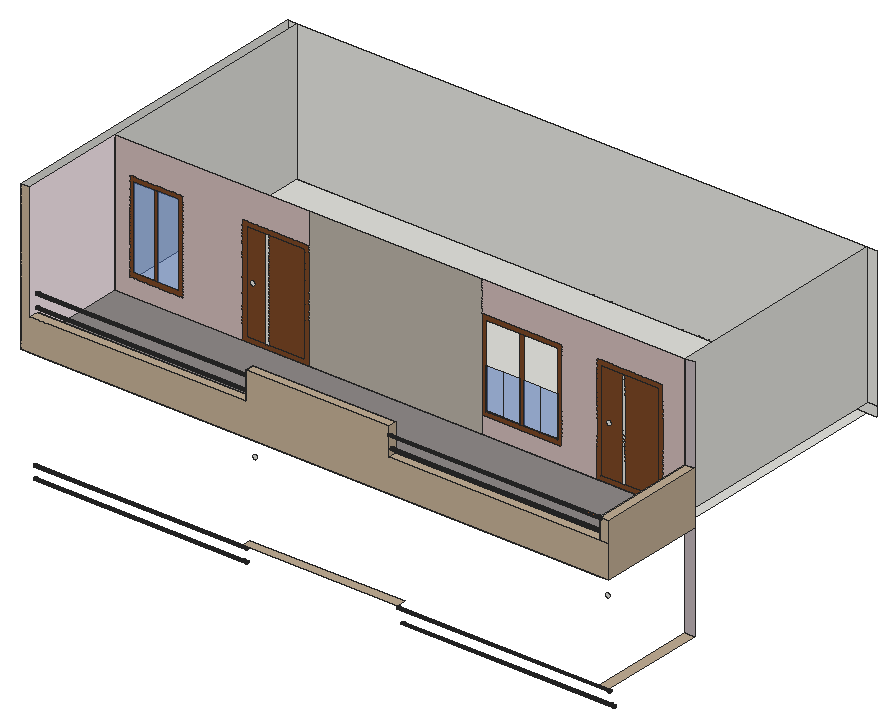
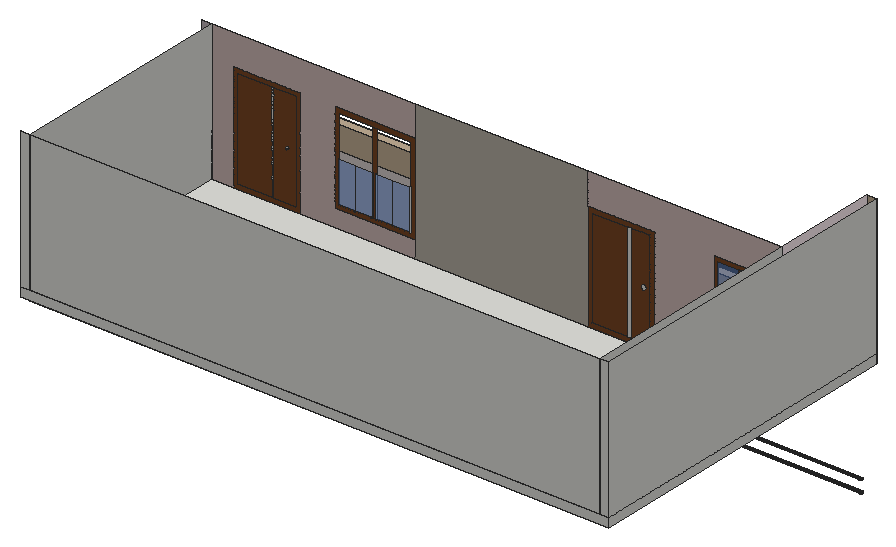
# SketchUp Ruby script. Lengths in inches.
U = 1.inch
M = Sketchup.active_model
def pt(a) = Geom::Point3d.new(a.map { |v| v * U })
def face(e, loops, mat)
  f = e.add_face(loops[0].map { |a| pt(a) })
  loops[1..].each { |l| e.add_face(l.map { |a| pt(a) }).erase! }
  f.material = f.back_material = mat if mat
  f
end
# faces: each face lists its corners as indices into pts; further lists are holes
def faces(e, pts, list, mat = nil) = list.each { |f| face(e, (f[0].is_a?(Array) ? f : [f]).map { |l| l.map { |i| pts[i] } }, mat) }
# xy, xz, yz: faces in a plane at the given z, y or x. An outline is a flat list of corners, or four numbers for a rectangle; further outlines are holes
def ring(l) = l.size == 4 ? [[l[0], l[1]], [l[2], l[1]], [l[2], l[3]], [l[0], l[3]]] : l.each_slice(2).to_a
def flat(e, list, mat, &to3) = list.each { |f| face(e, (f[0].is_a?(Array) ? f : [f]).map { |l| ring(l).map { |u, v| to3.(u, v) } }, mat) }
def xy(e, z, list, mat = nil) = flat(e, list, mat) { |x, y| [x, y, z] }
def xz(e, y, list, mat = nil) = flat(e, list, mat) { |x, z| [x, y, z] }
def yz(e, x, list, mat = nil) = flat(e, list, mat) { |y, z| [x, y, z] }
def lines(e, pts, list) = list.each { |a, b| e.add_line(pt(pts[a]), pt(pts[b])) }
# prism: a flat outline (further loops are holes) pulled along v
def prism(e, loops, v, mat = nil)
  f = face(e, loops, mat); d = Geom::Vector3d.new(v.map { |x| x * U })
  f.pushpull(f.normal.samedirection?(d) ? d.length : -d.length)
end
def box(e, o, s, mat = nil) = prism(e, [[o, [o[0] + s[0], o[1], o[2]], [o[0] + s[0], o[1] + s[1], o[2]], [o[0], o[1] + s[1], o[2]]]], [0, 0, s[2]], mat)
def at(x, y, z, deg = 0) = Geom::Transformation.translation(pt([x, y, z])) * Geom::Transformation.rotation(ORIGIN, Z_AXIS, deg.degrees)
def axes(o, x, y, z) = Geom::Transformation.new([*x, 0, *y, 0, *z, 0, *pt(o).to_a, 1])
def part(name) = M.definitions.add(name)
# library, detail: a bought-in or finely detailed component or shape, given as its bounding box
def library(name, o, s) = part(name).tap { |d| box(d.entities, o, s) }
def detail(e, o, s) = box(e.add_group.entities, o, s)
def put(e, d, t, mat = nil) = e.add_instance(d, t).tap { |i| i.material = mat if mat }
def group(e, t, mat = nil) = e.add_group.tap { |g| g.transformation = t; g.material = mat if mat }.entities
root = M.entities
M.materials.add("[0007_MistyRose]").color = [206, 184, 182]
M.materials.add("[0008_LavenderBlush]").color = [188, 177, 181]
M.materials.add("[0008_LavenderBlush]1").color = [255, 240, 245]
M.materials.add("[0012_Bisque]").color = [193, 173, 148]
M.materials.add("[0118_Thistle]").color = [198, 175, 198]
M.materials.add("[Stone Marble]").color = [143, 138, 136]
M.materials.add("[Stone Masonry Multi]").color = [182, 175, 164]
M.materials.add("[Translucent Glass Blue]").color = [100, 149, 237]
M.materials["[Translucent Glass Blue]"].alpha = 0.5
M.materials.add("[Wood Cherry Original]").color = [152, 86, 42]
M.materials.add("[Wood Veneer 01]").color = [120, 70, 37]
xy(root,900,[[574.875,12,976.5625,36],[1500,12,1524,288]],"[0012_Bisque]")
xy(root,1059.99,[[984.34,288,1028.68,289],[1028.68,288,1073.02,289],[1081.02,288,1125.36,289],[1125.36,288,1169.7,289]])
xy(root,1152,[[0,12,24,876],[24,288,1500,876]])
xy(root,1152,[[24,12,1500,288],[1500,12,1524,288]],"[0118_Thistle]")
xy(root,1176,[[24,288,1500,876]])
xy(root,1176,[[24,36,1500,288]],"[Stone Marble]")
xy(root,1232.18,[[984.34,288,1028.68,289],[1028.68,288,1073.02,289],[1081.02,288,1125.36,289],[1125.36,288,1169.7,289]])
xy(root,1236,[[24,12,582.625,36],[952.6875,12,1500,36]],"[0012_Bisque]")
xy(root,1290.02,[[1500,12,1524,288]],"[0012_Bisque]")
xy(root,1308,[[582.625,12,952.6875,36]],"[0012_Bisque]")
xz(root,12,[[0,1152,1524,1152,1524,1236,952.6875,1236,952.6875,1308,582.625,1308,582.625,1236,24,1236,24,1536,0,1536],[1500,1236,1524,1290.02]],"[0012_Bisque]")
xz(root,36,[[24,1176,24,1236,582.625,1236,582.625,1308,952.6875,1308,952.6875,1236,1500,1236,1500,1176]],"[0012_Bisque]")
xz(root,288,[[386.84,911.22,388.13,911.39,389.34,911.89,390.37,912.68,391.17,913.72,391.67,914.93,391.84,916.22,391.67,917.51,391.17,918.72,390.37,919.76,389.34,920.55,388.13,921.05,386.84,921.22,385.54,921.05,384.34,920.55,383.3,919.76,382.51,918.72,382.01,917.51,381.84,916.22,382.01,914.93,382.51,913.72,383.3,912.68,384.34,911.89,385.54,911.39],[1299.65,911.22,1300.94,911.39,1302.15,911.89,1303.18,912.68,1303.98,913.72,1304.48,914.93,1304.65,916.22,1304.48,917.51,1303.98,918.72,1303.18,919.76,1302.15,920.55,1300.94,921.05,1299.65,921.22,1298.35,921.05,1297.15,920.55,1296.11,919.76,1295.32,918.72,1294.82,917.51,1294.65,916.22,1294.82,914.93,1295.32,913.72,1296.11,912.68,1297.15,911.89,1298.35,911.39],[1500,1176,1524,1236],[415.26,1187.5,421.26,1444.49],[1338.64,1188,1344.64,1443.99],
  [1500,1236,1524,1290.02],[380.93,1312.17,382.22,1312.34,383.43,1312.84,384.46,1313.63,385.26,1314.67,385.76,1315.875,385.93,1317.17,385.76,1318.46,385.26,1319.67,384.46,1320.7,383.43,1321.5,382.22,1322,380.93,1322.17,379.63,1322,378.43,1321.5,377.39,1320.7,376.6,1319.67,376.1,1318.46,375.93,1317.17,376.1,1315.875,376.6,1314.67,377.39,1313.63,378.43,1312.84,379.63,1312.34],[1302.73,1312.17,1304.02,1312.34,1305.23,1312.84,1306.26,1313.63,1307.06,1314.67,1307.56,1315.875,1307.73,1317.17,1307.56,1318.46,1307.06,1319.67,1306.26,1320.7,1305.23,1321.5,1304.02,1322,1302.73,1322.17,1301.43,1322,1300.23,1321.5,1299.19,1320.7,1298.4,1319.67,1297.9,1318.46,1297.73,1317.17,1297.9,1315.875,1298.4,1314.67,1299.19,1313.63,1300.23,1312.84,1301.43,1312.34]])
xz(root,288,[[[24,1176,352.7,1176,352.7,1455.99,525.74,1455.99,525.74,1536,24,1536],[62.01,1220.68,200.45,1456.49]],[972.34,1176,1270.01,1176,1270.01,1455.99,1443.05,1455.99,1443.05,1176,1500,1176,1500,1536,972.34,1536,972.34,1455.99,1181.7,1455.99,1181.7,1220.18,972.34,1220.18]],"[0007_MistyRose]")
xz(root,288,[[1500,900,1524,1152],[1500,1290.02,1524,1536]],"[0008_LavenderBlush]")
xz(root,288,[[525.74,1176,972.34,1536]],"[Stone Masonry Multi]")
xz(root,288,[[74.01,1232.68,127.23,1444.49],[135.23,1232.68,188.45,1444.49]],"[Translucent Glass Blue]")
xz(root,288,[[[352.7,1176,525.74,1455.99],[364.2,1187.5,514.24,1444.49]],[[1270.01,1176,1443.05,1455.99],[1282.01,1188,1431.05,1443.99]],[[364.2,1187.5,415.26,1444.49],[380.93,1312.17,379.63,1312.34,378.43,1312.84,377.39,1313.63,376.6,1314.67,376.1,1315.875,375.93,1317.17,376.1,1318.46,376.6,1319.67,377.39,1320.7,378.43,1321.5,379.63,1322,380.93,1322.17,382.22,1322,383.43,1321.5,384.46,1320.7,385.26,1319.67,385.76,1318.46,385.93,1317.17,385.76,1315.875,385.26,1314.67,384.46,1313.63,383.43,1312.84,382.22,1312.34]],[421.26,1187.5,514.24,1444.49],[[1282.01,1188,1338.64,1443.99],[1302.73,1312.17,1301.43,1312.34,1300.23,1312.84,1299.19,1313.63,1298.4,1314.67,1297.9,1315.875,1297.73,1317.17,1297.9,1318.46,1298.4,1319.67,1299.19,1320.7,1300.23,1321.5,1301.43,1322,1302.73,1322.17,1304.02,1322,1305.23,1321.5,1306.26,1320.7,1307.06,1319.67,1307.56,1318.46,1307.73,1317.17,1307.56,1315.875,1307.06,1314.67,1306.26,1313.63,1305.23,1312.84,1304.02,1312.34]],
  [1344.64,1188,1431.05,1443.99],[[972.34,1220.18,1181.7,1455.99],[984.34,1232.18,1169.7,1443.99]],[[62.01,1220.68,200.45,1456.49],[74.01,1232.68,188.45,1444.49]],[1073.02,1232.18,1081.02,1443.99],[127.23,1232.68,135.23,1444.49]],"[Wood Veneer 01]")
xz(root,289,[[984.34,954.08,1028.68,1059.99],[1028.68,954.08,1073.02,1059.99],[1081.02,954.08,1125.36,1059.99],[1125.36,954.08,1169.7,1059.99],[984.34,1232.18,1028.68,1338.08],
  [1028.68,1232.18,1073.02,1338.08],[1081.02,1232.18,1125.36,1338.08],[1125.36,1232.18,1169.7,1338.08]],"[Translucent Glass Blue]")
xz(root,876,[[0,1152,1524,1176],[0,1176,24,1536],[24,1176,1500,1536],[1500,1176,1524,1536]])
yz(root,0,[[12,1152,876,1176],[12,1176,876,1536]])
yz(root,24,[[288,1176,876,1536]])
yz(root,24,[[36,1176,288,1176,288,1536,12,1536,12,1236,36,1236]],"[0008_LavenderBlush]1")
yz(root,582.625,[[12,1236,36,1308]])
yz(root,952.6875,[[13.5,1284.42,14.28,1284.52,15,1284.82,15.62,1285.3,16.1,1285.92,16.4,1286.65,16.5,1287.42,16.4,1288.2,16.1,1288.92,15.62,1289.54,15,1290.02,14.28,1290.32,13.5,1290.42,12.72,1290.32,12,1290.02,12,1284.82,12.72,1284.52]])
yz(root,952.6875,[[12,1236,36,1236,36,1308,12,1308,12,1290.02,12.72,1290.32,13.5,1290.42,14.28,1290.32,15,1290.02,15.62,1289.54,16.1,1288.92,16.4,1288.2,16.5,1287.42,16.4,1286.65,16.1,1285.92,15.62,1285.3,15,1284.82,14.28,1284.52,13.5,1284.42,12.72,1284.52,12,1284.82]],"[0012_Bisque]")
yz(root,984.34,[[288,954.08,289,1059.99],[288,1232.18,289,1338.08]])
yz(root,1073.02,[[288,954.08,289,1059.99],[288,1232.18,289,1338.08]])
yz(root,1081.02,[[288,954.08,289,1059.99],[288,1232.18,289,1338.08]])
yz(root,1169.7,[[288,954.08,289,1059.99],[288,1232.18,289,1338.08]])
yz(root,1500,[[288,1176,876,1536],[12,1236,36,1290.02]])
yz(root,1500,[[36,1176,288,1290.02]],"[0012_Bisque]")
yz(root,1524,[[12,1152,288,1290.02]],"[0012_Bisque]")
p = [[561.75,26.94,850.27],[24,26.94,850.27],[24,27.72,850.17],[561.75,27.72,850.17],[575.91,27.72,850.17],[575.91,26.94,850.27],
  [1513,26.94,850.27],[975.25,26.94,850.27],[975.25,27.72,850.17],[1513,27.72,850.17],[1527.16,27.72,850.17],[1527.16,26.94,850.27],
  [24,28.5,850.27],[561.75,28.5,850.27],[575.91,28.5,850.27],[975.25,28.5,850.27],[1513,28.5,850.27],[1527.16,28.5,850.27],
  [561.75,26.22,850.57],[24,26.22,850.57],[575.91,26.22,850.57],[1513,26.22,850.57],[975.25,26.22,850.57],[1527.16,26.22,850.57],
  [24,29.22,850.57],[561.75,29.22,850.57],[575.91,29.22,850.57],[975.25,29.22,850.57],[1513,29.22,850.57],[1527.16,29.22,850.57],
  [561.75,25.6,851.05],[24,25.6,851.05],[575.91,25.6,851.05],[1513,25.6,851.05],[975.25,25.6,851.05],[1527.16,25.6,851.05],
  [24,29.84,851.05],[561.75,29.84,851.05],[575.91,29.84,851.05],[975.25,29.84,851.05],[1513,29.84,851.05],[1527.16,29.84,851.05],
  [561.75,25.125,851.67],[24,25.125,851.67],[575.91,25.125,851.67],[1513,25.125,851.67],[975.25,25.125,851.67],[1527.16,25.125,851.67],
  [24,30.32,851.67],[561.75,30.32,851.67],[575.91,30.32,851.67],[975.25,30.32,851.67],[1513,30.32,851.67],[1527.16,30.32,851.67],
  [561.75,24.82,852.39],[24,24.82,852.39],[575.91,24.82,852.39],[1513,24.82,852.39],[975.25,24.82,852.39],[1527.16,24.82,852.39],
  [24,30.62,852.39],[561.75,30.62,852.39],[575.91,30.62,852.39],[975.25,30.62,852.39],[1513,30.62,852.39],[1527.16,30.62,852.39],
  [561.75,24.72,853.17],[24,24.72,853.17],[575.91,24.72,853.17],[1513,24.72,853.17],[975.25,24.72,853.17],[1527.16,24.72,853.17],
  [24,30.72,853.17],[561.75,30.72,853.17],[575.91,30.72,853.17],[975.25,30.72,853.17],[1513,30.72,853.17],[1527.16,30.72,853.17],
  [561.75,24.82,853.95],[24,24.82,853.95],[575.91,24.82,853.95],[1513,24.82,853.95],[975.25,24.82,853.95],[1527.16,24.82,853.95],
  [24,30.62,853.95],[561.75,30.62,853.95],[575.91,30.62,853.95],[975.25,30.62,853.95],[1513,30.62,853.95],[1527.16,30.62,853.95],
  [561.75,25.125,854.67],[24,25.125,854.67],[575.91,25.125,854.67],[1513,25.125,854.67],[975.25,25.125,854.67],[1527.16,25.125,854.67],
  [24,30.32,854.67],[561.75,30.32,854.67],[575.91,30.32,854.67],[975.25,30.32,854.67],[1513,30.32,854.67],[1527.16,30.32,854.67],
  [561.75,25.6,855.29],[24,25.6,855.29],[575.91,25.6,855.29],[1513,25.6,855.29],[975.25,25.6,855.29],[1527.16,25.6,855.29],
  [24,29.84,855.29],[561.75,29.84,855.29],[575.91,29.84,855.29],[975.25,29.84,855.29],[1513,29.84,855.29],[1527.16,29.84,855.29],
  [561.75,26.22,855.77],[24,26.22,855.77],[575.91,26.22,855.77],[1513,26.22,855.77],[975.25,26.22,855.77],[1527.16,26.22,855.77],
  [24,29.22,855.77],[561.75,29.22,855.77],[575.91,29.22,855.77],[975.25,29.22,855.77],[1513,29.22,855.77],[1527.16,29.22,855.77],
  [561.75,26.94,856.07],[24,26.94,856.07],[575.91,26.94,856.07],[1513,26.94,856.07],[975.25,26.94,856.07],[1527.16,26.94,856.07],
  [24,28.5,856.07],[561.75,28.5,856.07],[575.91,28.5,856.07],[975.25,28.5,856.07],[1513,28.5,856.07],[1527.16,28.5,856.07],
  [561.75,27.72,856.17],[24,27.72,856.17],[575.91,27.72,856.17],[1513,27.72,856.17],[975.25,27.72,856.17],[1527.16,27.72,856.17],
  [561.75,26.94,881.77],[24,26.94,881.77],[24,27.72,881.67],[561.75,27.72,881.67],[575.91,27.72,881.67],[575.91,26.94,881.77],
  [1501.1875,26.94,881.77],[963.4375,26.94,881.77],[963.4375,27.72,881.67],[1501.1875,27.72,881.67],[1515.34,27.72,881.67],[1515.34,26.94,881.77],
  [24,28.5,881.77],[561.75,28.5,881.77],[575.91,28.5,881.77],[963.4375,28.5,881.77],[1501.1875,28.5,881.77],[1515.34,28.5,881.77],
  [561.75,26.22,882.07],[24,26.22,882.07],[575.91,26.22,882.07],[1501.1875,26.22,882.07],[963.4375,26.22,882.07],[1515.34,26.22,882.07],
  [24,29.22,882.07],[561.75,29.22,882.07],[575.91,29.22,882.07],[963.4375,29.22,882.07],[1501.1875,29.22,882.07],[1515.34,29.22,882.07],
  [561.75,25.6,882.55],[24,25.6,882.55],[575.91,25.6,882.55],[1501.1875,25.6,882.55],[963.4375,25.6,882.55],[1515.34,25.6,882.55],
  [24,29.84,882.55],[561.75,29.84,882.55],[575.91,29.84,882.55],[963.4375,29.84,882.55],[1501.1875,29.84,882.55],[1515.34,29.84,882.55],
  [561.75,25.125,883.17],[24,25.125,883.17],[575.91,25.125,883.17],[1501.1875,25.125,883.17],[963.4375,25.125,883.17],[1515.34,25.125,883.17],
  [24,30.32,883.17],[561.75,30.32,883.17],[575.91,30.32,883.17],[963.4375,30.32,883.17],[1501.1875,30.32,883.17],[1515.34,30.32,883.17],
  [561.75,24.82,883.89],[24,24.82,883.89],[575.91,24.82,883.89],[1501.1875,24.82,883.89],[963.4375,24.82,883.89],[1515.34,24.82,883.89],
  [24,30.62,883.89],[561.75,30.62,883.89],[575.91,30.62,883.89],[963.4375,30.62,883.89],[1501.1875,30.62,883.89],[1515.34,30.62,883.89],
  [561.75,24.72,884.67],[24,24.72,884.67],[575.91,24.72,884.67],[1501.1875,24.72,884.67],[963.4375,24.72,884.67],[1515.34,24.72,884.67],
  [24,30.72,884.67],[561.75,30.72,884.67],[575.91,30.72,884.67],[963.4375,30.72,884.67],[1501.1875,30.72,884.67],[1515.34,30.72,884.67],
  [561.75,24.82,885.45],[24,24.82,885.45],[575.91,24.82,885.45],[1501.1875,24.82,885.45],[963.4375,24.82,885.45],[1515.34,24.82,885.45],
  [24,30.62,885.45],[561.75,30.62,885.45],[575.91,30.62,885.45],[963.4375,30.62,885.45],[1501.1875,30.62,885.45],[1515.34,30.62,885.45],
  [561.75,25.125,886.17],[24,25.125,886.17],[575.91,25.125,886.17],[1501.1875,25.125,886.17],[963.4375,25.125,886.17],[1515.34,25.125,886.17],
  [24,30.32,886.17],[561.75,30.32,886.17],[575.91,30.32,886.17],[963.4375,30.32,886.17],[1501.1875,30.32,886.17],[1515.34,30.32,886.17],
  [561.75,25.6,886.79],[24,25.6,886.79],[575.91,25.6,886.79],[1501.1875,25.6,886.79],[963.4375,25.6,886.79],[1515.34,25.6,886.79],
  [24,29.84,886.79],[561.75,29.84,886.79],[575.91,29.84,886.79],[963.4375,29.84,886.79],[1501.1875,29.84,886.79],[1515.34,29.84,886.79],
  [561.75,26.22,887.27],[24,26.22,887.27],[575.91,26.22,887.27],[1501.1875,26.22,887.27],[963.4375,26.22,887.27],[1515.34,26.22,887.27],
  [24,29.22,887.27],[561.75,29.22,887.27],[575.91,29.22,887.27],[963.4375,29.22,887.27],[1501.1875,29.22,887.27],[1515.34,29.22,887.27],
  [561.75,26.94,887.57],[24,26.94,887.57],[575.91,26.94,887.57],[1501.1875,26.94,887.57],[963.4375,26.94,887.57],[1515.34,26.94,887.57],
  [24,28.5,887.57],[561.75,28.5,887.57],[575.91,28.5,887.57],[963.4375,28.5,887.57],[1501.1875,28.5,887.57],[1515.34,28.5,887.57],
  [561.75,27.72,887.67],[24,27.72,887.67],[575.91,27.72,887.67],[1501.1875,27.72,887.67],[963.4375,27.72,887.67],[1515.34,27.72,887.67],
  [567.75,26.22,1249.35],[30,26.22,1249.35],[30,27,1249.25],[567.75,27,1249.25],[581.91,27,1249.25],[581.91,26.22,1249.35],
  [30,27.78,1249.35],[567.75,27.78,1249.35],[581.91,27.78,1249.35],[567.75,25.5,1249.65],[30,25.5,1249.65],[581.91,25.5,1249.65],
  [30,28.5,1249.65],[567.75,28.5,1249.65],[581.91,28.5,1249.65],[567.75,24.88,1250.13],[30,24.88,1250.13],[581.91,24.88,1250.13],
  [30,29.12,1250.13],[567.75,29.12,1250.13],[581.91,29.12,1250.13],[567.75,24.4,1250.75],[30,24.4,1250.75],[581.91,24.4,1250.75],
  [30,29.6,1250.75],[567.75,29.6,1250.75],[581.91,29.6,1250.75],[567.75,24.1,1251.47],[30,24.1,1251.47],[581.91,24.1,1251.47],
  [30,29.9,1251.47],[567.75,29.9,1251.47],[581.91,29.9,1251.47],[1490.4375,18.09,1251.08],[952.6875,18.09,1251.08],[952.6875,18.87,1250.98],
  [1490.4375,18.87,1250.98],[1504.59,18.87,1250.98],[1504.59,18.09,1251.08],[952.6875,19.65,1251.08],[1490.4375,19.65,1251.08],[1504.59,19.65,1251.08],
  [1490.4375,17.37,1251.38],[952.6875,17.37,1251.38],[1504.59,17.37,1251.38],[952.6875,20.37,1251.38],[1490.4375,20.37,1251.38],[1504.59,20.37,1251.38],
  [1490.4375,16.75,1251.86],[952.6875,16.75,1251.86],[1504.59,16.75,1251.86],[952.6875,20.99,1251.86],[1490.4375,20.99,1251.86],[1504.59,20.99,1251.86],
  [567.75,24,1252.25],[30,24,1252.25],[581.91,24,1252.25],[30,30,1252.25],[567.75,30,1252.25],[581.91,30,1252.25],
  [1490.4375,16.27,1252.48],[952.6875,16.27,1252.48],[1504.59,16.27,1252.48],[952.6875,21.47,1252.48],[1490.4375,21.47,1252.48],[1504.59,21.47,1252.48],
  [567.75,24.1,1253.03],[30,24.1,1253.03],[581.91,24.1,1253.03],[30,29.9,1253.03],[567.75,29.9,1253.03],[581.91,29.9,1253.03],
  [1490.4375,15.97,1253.21],[952.6875,15.97,1253.21],[1504.59,15.97,1253.21],[952.6875,21.77,1253.21],[1490.4375,21.77,1253.21],[1504.59,21.77,1253.21],
  [567.75,24.4,1253.75],[30,24.4,1253.75],[581.91,24.4,1253.75],[30,29.6,1253.75],[567.75,29.6,1253.75],[581.91,29.6,1253.75],
  [1490.4375,15.87,1253.98],[952.6875,15.87,1253.98],[1504.59,15.87,1253.98],[952.6875,21.87,1253.98],[1490.4375,21.87,1253.98],[1504.59,21.87,1253.98],
  [567.75,24.88,1254.37],[30,24.88,1254.37],[581.91,24.88,1254.37],[30,29.12,1254.37],[567.75,29.12,1254.37],[581.91,29.12,1254.37],
  [1490.4375,15.97,1254.76],[952.6875,15.97,1254.76],[1504.59,15.97,1254.76],[952.6875,21.77,1254.76],[1490.4375,21.77,1254.76],[1504.59,21.77,1254.76],
  [567.75,25.5,1254.85],[30,25.5,1254.85],[581.91,25.5,1254.85],[30,28.5,1254.85],[567.75,28.5,1254.85],[581.91,28.5,1254.85],
  [1490.4375,16.27,1255.48],[952.6875,16.27,1255.48],[1504.59,16.27,1255.48],[952.6875,21.47,1255.48],[1490.4375,21.47,1255.48],[1504.59,21.47,1255.48],
  [567.75,26.22,1255.15],[30,26.22,1255.15],[581.91,26.22,1255.15],[30,27.78,1255.15],[567.75,27.78,1255.15],[581.91,27.78,1255.15],
  [567.75,27,1255.25],[30,27,1255.25],[581.91,27,1255.25],[1490.4375,16.75,1256.1],[952.6875,16.75,1256.1],[1504.59,16.75,1256.1],
  [952.6875,20.99,1256.1],[1490.4375,20.99,1256.1],[1504.59,20.99,1256.1],[1490.4375,17.37,1256.58],[952.6875,17.37,1256.58],[1504.59,17.37,1256.58],
  [952.6875,20.37,1256.58],[1490.4375,20.37,1256.58],[1504.59,20.37,1256.58],[1490.4375,18.09,1256.88],[952.6875,18.09,1256.88],[1504.59,18.09,1256.88],
  [952.6875,19.65,1256.88],[1490.4375,19.65,1256.88],[1504.59,19.65,1256.88],[1490.4375,18.87,1256.98],[952.6875,18.87,1256.98],[1504.59,18.87,1256.98],
  [567.75,26.22,1282.85],[30,26.22,1282.85],[30,27,1282.75],[567.75,27,1282.75],[581.91,27,1282.75],[581.91,26.22,1282.85],
  [30,27.78,1282.85],[567.75,27.78,1282.85],[581.91,27.78,1282.85],[567.75,25.5,1283.15],[30,25.5,1283.15],[581.91,25.5,1283.15],
  [30,28.5,1283.15],[567.75,28.5,1283.15],[581.91,28.5,1283.15],[567.75,24.88,1283.63],[30,24.88,1283.63],[581.91,24.88,1283.63],
  [30,29.12,1283.63],[567.75,29.12,1283.63],[581.91,29.12,1283.63],[567.75,24.4,1284.25],[30,24.4,1284.25],[581.91,24.4,1284.25],
  [30,29.6,1284.25],[567.75,29.6,1284.25],[581.91,29.6,1284.25],[567.75,24.1,1284.97],[30,24.1,1284.97],[581.91,24.1,1284.97],
  [30,29.9,1284.97],[567.75,29.9,1284.97],[581.91,29.9,1284.97],[1490.4375,12.72,1284.52],[952.6875,12.72,1284.52],[952.6875,13.5,1284.42],
  [1490.4375,13.5,1284.42],[1504.59,13.5,1284.42],[1504.59,12.72,1284.52],[952.6875,14.28,1284.52],[1490.4375,14.28,1284.52],[1504.59,14.28,1284.52],
  [1490.4375,12,1284.82],[952.6875,12,1284.82],[1504.59,12,1284.82],[1500,12,1284.82],[952.6875,15,1284.82],[1490.4375,15,1284.82],
  [1504.59,15,1284.82],[1490.4375,11.38,1285.3],[952.6875,11.38,1285.3],[1504.59,11.38,1285.3],[952.6875,15.62,1285.3],[1490.4375,15.62,1285.3],
  [1504.59,15.62,1285.3],[567.75,24,1285.75],[30,24,1285.75],[581.91,24,1285.75],[30,30,1285.75],[567.75,30,1285.75],
  [581.91,30,1285.75],[1490.4375,10.9,1285.92],[952.6875,10.9,1285.92],[1504.59,10.9,1285.92],[952.6875,16.1,1285.92],[1490.4375,16.1,1285.92],
  [1504.59,16.1,1285.92],[567.75,24.1,1286.53],[30,24.1,1286.53],[581.91,24.1,1286.53],[30,29.9,1286.53],[567.75,29.9,1286.53],
  [581.91,29.9,1286.53],[1490.4375,10.6,1286.65],[952.6875,10.6,1286.65],[1504.59,10.6,1286.65],[952.6875,16.4,1286.65],[1490.4375,16.4,1286.65],
  [1504.59,16.4,1286.65],[567.75,24.4,1287.25],[30,24.4,1287.25],[581.91,24.4,1287.25],[30,29.6,1287.25],[567.75,29.6,1287.25],
  [581.91,29.6,1287.25],[1490.4375,10.5,1287.42],[952.6875,10.5,1287.42],[1504.59,10.5,1287.42],[952.6875,16.5,1287.42],[1490.4375,16.5,1287.42],
  [1504.59,16.5,1287.42],[567.75,24.88,1287.87],[30,24.88,1287.87],[581.91,24.88,1287.87],[30,29.12,1287.87],[567.75,29.12,1287.87],
  [581.91,29.12,1287.87],[1490.4375,10.6,1288.2],[952.6875,10.6,1288.2],[1504.59,10.6,1288.2],[952.6875,16.4,1288.2],[1490.4375,16.4,1288.2],
  [1504.59,16.4,1288.2],[567.75,25.5,1288.35],[30,25.5,1288.35],[581.91,25.5,1288.35],[30,28.5,1288.35],[567.75,28.5,1288.35],
  [581.91,28.5,1288.35],[1490.4375,10.9,1288.92],[952.6875,10.9,1288.92],[1504.59,10.9,1288.92],[952.6875,16.1,1288.92],[1490.4375,16.1,1288.92],
  [1504.59,16.1,1288.92],[567.75,26.22,1288.65],[30,26.22,1288.65],[581.91,26.22,1288.65],[30,27.78,1288.65],[567.75,27.78,1288.65],
  [581.91,27.78,1288.65],[567.75,27,1288.75],[30,27,1288.75],[581.91,27,1288.75],[1490.4375,11.38,1289.54],[952.6875,11.38,1289.54],
  [1504.59,11.38,1289.54],[952.6875,15.62,1289.54],[1490.4375,15.62,1289.54],[1504.59,15.62,1289.54],[1490.4375,12,1290.02],[952.6875,12,1290.02],
  [1504.59,12,1290.02],[1500,12,1290.02],[952.6875,15,1290.02],[1490.4375,15,1290.02],[1500,15,1290.02],[1504.59,15,1290.02],
  [1490.4375,12.72,1290.32],[952.6875,12.72,1290.32],[1504.59,12.72,1290.32],[952.6875,14.28,1290.32],[1490.4375,14.28,1290.32],[1504.59,14.28,1290.32],
  [1490.4375,13.5,1290.42],[952.6875,13.5,1290.42],[1504.59,13.5,1290.42]]
faces(root,p,[[0,1,2,3,4,5],[6,7,8,9,10,11],[3,2,12,13,14,4],[9,8,15,16,17,10],[18,19,1,0,5,20],[21,22,7,6,11,23],[13,12,24,25,26,14],[16,15,27,28,29,17],
  [30,31,19,18,20,32],[33,34,22,21,23,35],[25,24,36,37,38,26],[28,27,39,40,41,29],[42,43,31,30,32,44],[45,46,34,33,35,47],[37,36,48,49,50,38],[40,39,51,52,53,41],
  [54,55,43,42,44,56],[57,58,46,45,47,59],[49,48,60,61,62,50],[52,51,63,64,65,53],[66,67,55,54,56,68],[69,70,58,57,59,71],[61,60,72,73,74,62],[64,63,75,76,77,65],
  [78,79,67,66,68,80],[81,82,70,69,71,83],[73,72,84,85,86,74],[76,75,87,88,89,77],[90,91,79,78,80,92],[93,94,82,81,83,95],[85,84,96,97,98,86],[88,87,99,100,101,89],
  [102,103,91,90,92,104],[105,106,94,93,95,107],[97,96,108,109,110,98],[100,99,111,112,113,101],[114,115,103,102,104,116],[117,118,106,105,107,119],[109,108,120,121,122,110],[112,111,123,124,125,113],
  [126,127,115,114,116,128],[129,130,118,117,119,131],[121,120,132,133,134,122],[124,123,135,136,137,125],[138,139,127,126,128,140],[141,142,130,129,131,143],[133,132,139,138,140,134],[136,135,142,141,143,137],
  [144,145,146,147,148,149],[150,151,152,153,154,155],[147,146,156,157,158,148],[153,152,159,160,161,154],[162,163,145,144,149,164],[165,166,151,150,155,167],[157,156,168,169,170,158],[160,159,171,172,173,161],
  [174,175,163,162,164,176],[177,178,166,165,167,179],[169,168,180,181,182,170],[172,171,183,184,185,173],[186,187,175,174,176,188],[189,190,178,177,179,191],[181,180,192,193,194,182],[184,183,195,196,197,185],
  [198,199,187,186,188,200],[201,202,190,189,191,203],[193,192,204,205,206,194],[196,195,207,208,209,197],[210,211,199,198,200,212],[213,214,202,201,203,215],[205,204,216,217,218,206],[208,207,219,220,221,209],
  [222,223,211,210,212,224],[225,226,214,213,215,227],[217,216,228,229,230,218],[220,219,231,232,233,221],[234,235,223,222,224,236],[237,238,226,225,227,239],[229,228,240,241,242,230],[232,231,243,244,245,233],
  [246,247,235,234,236,248],[249,250,238,237,239,251],[241,240,252,253,254,242],[244,243,255,256,257,245],[258,259,247,246,248,260],[261,262,250,249,251,263],[253,252,264,265,266,254],[256,255,267,268,269,257],
  [270,271,259,258,260,272],[273,274,262,261,263,275],[265,264,276,277,278,266],[268,267,279,280,281,269],[282,283,271,270,272,284],[285,286,274,273,275,287],[277,276,283,282,284,278],[280,279,286,285,287,281],
  [288,289,290,291,292,293],[291,290,294,295,296,292],[297,298,289,288,293,299],[295,294,300,301,302,296],[303,304,298,297,299,305],[301,300,306,307,308,302],[309,310,304,303,305,311],[307,306,312,313,314,308],
  [315,316,310,309,311,317],[313,312,318,319,320,314],[321,322,323,324,325,326],[324,323,327,328,329,325],[330,331,322,321,326,332],[328,327,333,334,335,329],[336,337,331,330,332,338],[334,333,339,340,341,335],
  [342,343,316,315,317,344],[319,318,345,346,347,320],[348,349,337,336,338,350],[340,339,351,352,353,341],[354,355,343,342,344,356],[346,345,357,358,359,347],[360,361,349,348,350,362],[352,351,363,364,365,353],
  [366,367,355,354,356,368],[358,357,369,370,371,359],[372,373,361,360,362,374],[364,363,375,376,377,365],[378,379,367,366,368,380],[370,369,381,382,383,371],[384,385,373,372,374,386],[376,375,387,388,389,377],
  [390,391,379,378,380,392],[382,381,393,394,395,383],[396,397,385,384,386,398],[388,387,399,400,401,389],[402,403,391,390,392,404],[394,393,405,406,407,395],[408,409,403,402,404,410],[406,405,409,408,410,407],
  [411,412,397,396,398,413],[400,399,414,415,416,401],[417,418,412,411,413,419],[415,414,420,421,422,416],[423,424,418,417,419,425],[421,420,426,427,428,422],[429,430,424,423,425,431],[427,426,430,429,431,428],
  [432,433,434,435,436,437],[435,434,438,439,440,436],[441,442,433,432,437,443],[439,438,444,445,446,440],[447,448,442,441,443,449],[445,444,450,451,452,446],[453,454,448,447,449,455],[451,450,456,457,458,452],
  [459,460,454,453,455,461],[457,456,462,463,464,458],[465,466,467,468,469,470],[468,467,471,472,473,469],[474,475,466,465,470,476,477],[472,471,478,479,480,473],[481,482,475,474,477,476,483],[479,478,484,485,486,480],
  [487,488,460,459,461,489],[463,462,490,491,492,464],[493,494,482,481,483,495],[485,484,496,497,498,486],[499,500,488,487,489,501],[491,490,502,503,504,492],[505,506,494,493,495,507],[497,496,508,509,510,498],
  [511,512,500,499,501,513],[503,502,514,515,516,504],[517,518,506,505,507,519],[509,508,520,521,522,510],[523,524,512,511,513,525],[515,514,526,527,528,516],[529,530,518,517,519,531],[521,520,532,533,534,522],
  [535,536,524,523,525,537],[527,526,538,539,540,528],[541,542,530,529,531,543],[533,532,544,545,546,534],[547,548,536,535,537,549],[539,538,550,551,552,540],[553,554,548,547,549,555],[551,550,554,553,555,552],
  [556,557,542,541,543,558],[545,544,559,560,561,546],[562,563,557,556,558,564,565],[560,559,566,567,568,569,561],[570,571,563,562,565,564,572],[567,566,573,574,575,569,568],[576,577,571,570,572,578],[574,573,577,576,578,575]],"[Wood Cherry Original]")
